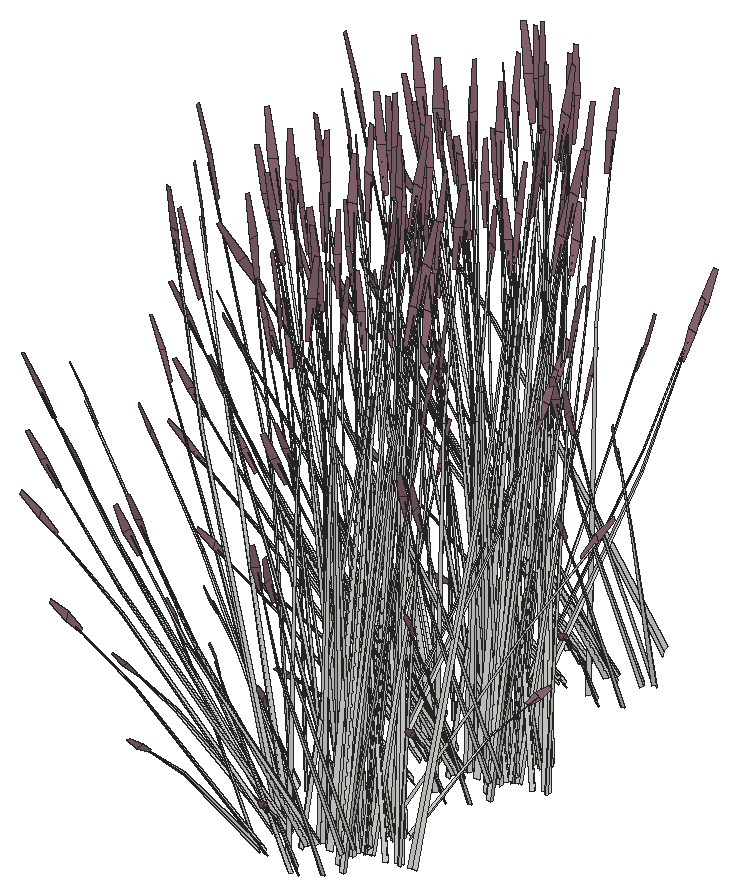
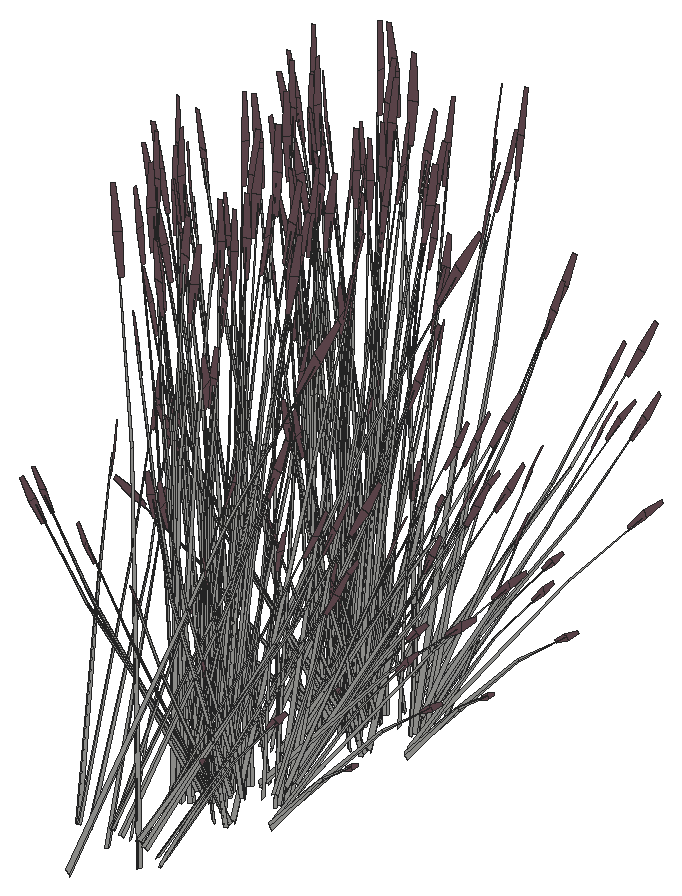
# SketchUp Ruby script. Lengths in inches.
U = 1.inch
M = Sketchup.active_model
def pt(a) = Geom::Point3d.new(a.map { |v| v * U })
def face(e, loops, mat)
  f = e.add_face(loops[0].map { |a| pt(a) })
  loops[1..].each { |l| e.add_face(l.map { |a| pt(a) }).erase! }
  f.material = f.back_material = mat if mat
  f
end
# faces: each face lists its corners as indices into pts; further lists are holes
def faces(e, pts, list, mat = nil) = list.each { |f| face(e, (f[0].is_a?(Array) ? f : [f]).map { |l| l.map { |i| pts[i] } }, mat) }
# xy, xz, yz: faces in a plane at the given z, y or x. An outline is a flat list of corners, or four numbers for a rectangle; further outlines are holes
def ring(l) = l.size == 4 ? [[l[0], l[1]], [l[2], l[1]], [l[2], l[3]], [l[0], l[3]]] : l.each_slice(2).to_a
def flat(e, list, mat, &to3) = list.each { |f| face(e, (f[0].is_a?(Array) ? f : [f]).map { |l| ring(l).map { |u, v| to3.(u, v) } }, mat) }
def xy(e, z, list, mat = nil) = flat(e, list, mat) { |x, y| [x, y, z] }
def xz(e, y, list, mat = nil) = flat(e, list, mat) { |x, z| [x, y, z] }
def yz(e, x, list, mat = nil) = flat(e, list, mat) { |y, z| [x, y, z] }
def lines(e, pts, list) = list.each { |a, b| e.add_line(pt(pts[a]), pt(pts[b])) }
# prism: a flat outline (further loops are holes) pulled along v
def prism(e, loops, v, mat = nil)
  f = face(e, loops, mat); d = Geom::Vector3d.new(v.map { |x| x * U })
  f.pushpull(f.normal.samedirection?(d) ? d.length : -d.length)
end
def box(e, o, s, mat = nil) = prism(e, [[o, [o[0] + s[0], o[1], o[2]], [o[0] + s[0], o[1] + s[1], o[2]], [o[0], o[1] + s[1], o[2]]]], [0, 0, s[2]], mat)
def at(x, y, z, deg = 0) = Geom::Transformation.translation(pt([x, y, z])) * Geom::Transformation.rotation(ORIGIN, Z_AXIS, deg.degrees)
def axes(o, x, y, z) = Geom::Transformation.new([*x, 0, *y, 0, *z, 0, *pt(o).to_a, 1])
def part(name) = M.definitions.add(name)
# library, detail: a bought-in or finely detailed component or shape, given as its bounding box
def library(name, o, s) = part(name).tap { |d| box(d.entities, o, s) }
def detail(e, o, s) = box(e.add_group.entities, o, s)
def put(e, d, t, mat = nil) = e.add_instance(d, t).tap { |i| i.material = mat if mat }
def group(e, t, mat = nil) = e.add_group.tap { |g| g.transformation = t; g.material = mat if mat }.entities
root = M.entities
M.materials.add("LightPink_Translucent").color = [144, 107, 117]
c1 = part("blade")
p = [[2.15,0.21,22],[0,0.17,0],[0.09,0.45,0],[2.18,0.31,22],[2.29,0.31,22],[0.38,0.45,0],
  [2.48,0.24,33],[2.49,0.24,33],[2.48,0.22,33]]
faces(c1.entities,p,[[0,1,2,3],[4,5,2,3],[6,3,4,7],[8,0,3,6]])
c2 = part("seeds")
p = [[0.3,-0.1,1.38],[-0.01,-0.03,1.59],[-0.01,-0.03,0.03],[0.14,-0.07,-0.07],[0.29,-0.03,3],[0.15,0.01,3.11]]
faces(c2.entities,p,[[0,1,2,3],[1,0,4,5]],"LightPink_Translucent")
c3 = part("blade with seeds")
put(c3.entities,c1,at(0,0,0))
put(c3.entities,c2,axes([2.4,0.25,30.99],[1.5799,-0.05474,1.17369],[-0.12525,1.92788,0.29478],[-0.07173,-0.02425,1.56792]))
put(root,c3,axes([23.83,24.14,44.84],[0.42589,0.08502,1.43002],[0.2745,0.86839,-0.30754],[-0.57851,0.16255,0.61141]))
put(root,c3,axes([26.46,19.68,47.23],[-1.22504,-0.02494,-0.71045],[0.08228,-1.05005,0.08574],[-0.51899,-0.11081,1.00501]))
put(root,c3,axes([25.48,19.94,44.84],[0.23927,0.28834,1.43002],[-0.55135,0.78376,-0.30754],[-0.56612,-0.18733,0.61141]))
put(root,c3,axes([25.375,40.2,44.59],[0.42589,0.08502,1.43002],[0.2745,0.86839,-0.30754],[-0.57851,0.16255,0.61141]))
put(root,c3,axes([29.14,37.42,45.34],[0.34834,-0.14982,1.77064],[0.12012,1.04605,0.13857],[-0.75452,0.1388,0.63284]))
put(root,c3,axes([25.19,21.93,46.93],[-0.332,0.94205,-0.51099],[-1.13828,-0.3229,-0.3958],[-0.45829,0.08638,0.97773]))
put(root,c3,axes([26.06,19.9,46.93],[-0.88986,0.68603,-0.51099],[-0.77932,-0.72471,-0.3958],[-0.45212,-0.10438,0.97773]))
put(root,c3,axes([28.01,35.75,46.98],[-1.22504,-0.02494,-0.71045],[0.08228,-1.05005,0.08574],[-0.51899,-0.11081,1.00501]))
put(root,c3,axes([27.02,36,44.59],[0.23927,0.28834,1.43002],[-0.55135,0.78376,-0.30754],[-0.56612,-0.18733,0.61141]))
put(root,c3,axes([22.94,25.96,45.02],[0.51072,-0.46938,1.1486],[0.20153,0.74307,0.84392],[-0.36908,0.13305,0.25299]))
put(root,c3,axes([26.04,37.5625,46.53],[-1.01846,-0.28891,-0.35414],[0.29705,-0.84289,0.4572],[-0.41005,0.07729,0.87481]))
put(root,c3,axes([26.74,37.99,46.68],[-0.332,0.94205,-0.51099],[-1.13828,-0.3229,-0.3958],[-0.45829,0.08638,0.97773]))
put(root,c3,axes([27.6,35.96,46.68],[-0.88986,0.68603,-0.51099],[-0.77932,-0.72471,-0.3958],[-0.45212,-0.10438,0.97773]))
put(root,c3,axes([24.05,20.81,45.02],[0.78239,-0.07411,1.1486],[-0.49629,0.65296,0.84392],[-0.38663,-0.09795,0.25299]))
put(root,c3,axes([24.49,42.02,44.77],[0.51072,-0.46938,1.1486],[0.20153,0.74307,0.84392],[-0.36908,0.13305,0.25299]))
put(root,c3,axes([26.97,54.34,46.53],[-0.69728,-0.64842,-0.35414],[0.79619,-0.61382,0.4572],[-0.40453,-0.09339,0.87481]))
put(root,c3,axes([27.27,35.3125,46.53],[-0.69728,-0.64842,-0.35414],[0.79619,-0.61382,0.4572],[-0.40453,-0.09339,0.87481]))
put(root,c3,axes([26.41,39.99,46.53],[-1.06674,0.14801,-0.35414],[-0.28168,-0.84611,0.4572],[-0.30569,0.22726,0.87481]))
put(root,c3,axes([25.6,36.87,44.77],[0.78239,-0.07411,1.1486],[-0.49629,0.65296,0.84392],[-0.38663,-0.09795,0.25299]))
put(root,c3,axes([25.75,24.03,46.93],[0.31482,0.94565,-0.51099],[-1.19224,0.16542,-0.3958],[-0.34166,0.254,0.97773]))
put(root,c3,axes([28.59,18.45,47.23],[-1.04497,-0.50058,-0.71045],[0.74264,-0.8772,0.08574],[-0.3786,-0.29889,1.00501]))
put(root,c3,axes([28.11,18.47,46.93],[-1.20928,0.24619,-0.51099],[-0.21154,-0.93233,-0.3958],[-0.32481,-0.26718,0.97773]))
put(root,c3,axes([27.75,25.96,44.625],[-0.7662,1.03778,0],[-1.28187,-0.57875,-0.51607],[-0.29196,-0.13181,1.63711]))
put(root,c3,axes([27.29,40.09,46.68],[0.31482,0.94565,-0.51099],[-1.19224,0.16542,-0.3958],[-0.34166,0.254,0.97773]))
put(root,c3,axes([29.84,53.54,46.98],[-1.04497,-0.50058,-0.71045],[0.74264,-0.8772,0.08574],[-0.3786,-0.29889,1.00501]))
put(root,c3,axes([29.35,53.5625,46.68],[-1.20928,0.24619,-0.51099],[-0.21154,-0.93233,-0.3958],[-0.32481,-0.26718,0.97773]))
put(root,c3,axes([30.14,34.51,46.98],[-1.04497,-0.50058,-0.71045],[0.74264,-0.8772,0.08574],[-0.3786,-0.29889,1.00501]))
put(root,c3,axes([26.35,27.46,44.84],[0.38672,-0.16338,1.43002],[0.95481,0.49262,-0.30754],[-0.28419,0.42626,0.61141]))
put(root,c3,axes([29.65,34.53,46.68],[-1.20928,0.24619,-0.51099],[-0.21154,-0.93233,-0.3958],[-0.32481,-0.26718,0.97773]))
put(root,c3,axes([25.8,18.15,44.38],[-0.35352,0.84566,-0.03893],[-1.08806,-0.26014,-0.17649],[-0.1652,-0.13832,0.58215]))
put(root,c3,axes([27.43,17.08,44.84],[-0.07421,0.33879,1.43002],[-1.08488,0.28361,-0.30754],[-0.25359,-0.4379,0.61141]))
put(root,c3,axes([29.29,42.02,44.375],[-0.7662,1.03778,0],[-1.28187,-0.57875,-0.51607],[-0.29196,-0.13181,1.63711]))
put(root,c3,axes([25.22,22.01,44.625],[-1.53239,0,0],[0,-1.1575,-0.51607],[0,-0.26363,1.63711]))
put(root,c3,axes([27.89,43.52,44.59],[0.38672,-0.16338,1.43002],[0.95481,0.49262,-0.30754],[-0.28419,0.42626,0.61141]))
put(root,c3,axes([28.67,52.17,44.59],[-0.07421,0.33879,1.43002],[-1.08488,0.28361,-0.30754],[-0.25359,-0.4379,0.61141]))
put(root,c3,axes([26.4,21.7,44.58],[-1.1399,0.87071,0.30756],[-1.1406,-0.86155,-0.36492],[-0.03981,-0.24727,1.64885]))
put(root,c3,axes([28.97,33.14,44.59],[-0.07421,0.33879,1.43002],[-1.08488,0.28361,-0.30754],[-0.25359,-0.4379,0.61141]))
put(root,c3,axes([29.48,52.875,46.53],[-0.18927,-0.83419,-0.35414],[1.08199,-0.22027,0.4572],[-0.29062,-0.23905,0.87481]))
put(root,c3,axes([27.05,16.54,45.02],[0.63926,0.36046,1.1486],[-0.93099,0.21668,0.84392],[-0.1992,-0.27702,0.25299]))
put(root,c3,axes([27.3,25.32,47.59],[-0.03189,0.95798,-0.7886],[-1.34277,-0.06434,0.09517],[-0.14171,0.40585,1.11556]))
put(root,c3,axes([29.78,33.84,46.53],[-0.18927,-0.83419,-0.35414],[1.08199,-0.22027,0.4572],[-0.29062,-0.23905,0.87481]))
put(root,c3,axes([26.76,38.07,44.375],[-1.53239,0,0],[0,-1.1575,-0.51607],[0,-0.26363,1.63711]))
put(root,c3,axes([27.27,28.01,45.02],[-0.03171,-0.6158,1.1486],[0.7925,0.43922,0.84392],[-0.15586,0.29352,0.25299]))
put(root,c3,axes([28.29,41.95,46.53],[-0.82919,0.54528,-0.35414],[-0.78493,-0.62262,0.4572],[-0.11943,0.31634,0.87481]))
put(root,c3,axes([28.41,25.42,44.73],[1.14694,0.51783,0.49651],[-0.68554,0.92854,0],[-0.26122,-0.11794,1.57504]))
put(root,c3,axes([32.34,59.2,45.33],[1.05902,0.41762,1.51261],[-1.03748,0.89969,0.59816],[-0.46471,-0.53324,1.26806]))
put(root,c3,axes([27.95,37.76,44.33],[-1.1399,0.87071,0.30756],[-1.1406,-0.86155,-0.36492],[-0.03981,-0.24727,1.64885]))
put(root,c3,axes([29.49,23.52,44.69],[0.32481,-1.2272,-0.23429],[1.54007,0.21392,0.51271],[-0.26911,-0.16947,1.5644]))
put(root,c3,axes([28.3,51.625,44.77],[0.63926,0.36046,1.1486],[-0.93099,0.21668,0.84392],[-0.1992,-0.27702,0.25299]))
put(root,c3,axes([32.64,40.17,45.33],[1.05902,0.41762,1.51261],[-1.03748,0.89969,0.59816],[-0.46471,-0.53324,1.26806]))
put(root,c3,axes([30.05,23.81,44.87],[-0.23642,0.92427,0.1448],[-1.15506,-0.16044,-0.41347],[-0.21021,-0.09491,1.26744]))
put(root,c3,axes([28.6,32.6,44.77],[0.63926,0.36046,1.1486],[-0.93099,0.21668,0.84392],[-0.1992,-0.27702,0.25299]))
put(root,c3,axes([26.15,22.18,44.73],[0,1.03566,0.49651],[-1.37109,0,0],[0,-0.23588,1.57504]))
put(root,c3,axes([32.43,26.11,44.44],[-0.75665,-1.04141,-0.05142],[1.28187,-0.57875,0.51607],[-0.31588,0.09915,1.6363]))
put(root,c3,axes([28.84,41.375,47.34],[-0.03189,0.95798,-0.7886],[-1.34277,-0.06434,0.09517],[-0.14171,0.40585,1.11556]))
put(root,c3,axes([28.82,44.07,44.77],[-0.03171,-0.6158,1.1486],[0.7925,0.43922,0.84392],[-0.15586,0.29352,0.25299]))
put(root,c3,axes([27.57,25.63,47.26],[0.87728,0.69587,-0.5672],[-0.92674,0.60943,-0.43934],[-0.13348,0.35356,1.08528]))
put(root,c3,axes([32.74,22.11,45.09],[-0.03348,-0.97511,1.41272],[1.51511,0.25277,0.59816],[-0.35835,0.53357,1.3335]))
put(root,c3,axes([29.95,41.48,44.48],[1.14694,0.51783,0.49651],[-0.68554,0.92854,0],[-0.26122,-0.11794,1.57504]))
put(root,c3,axes([26.62,26.68,45.07],[1.11329,-0.1834,0.06507],[0.25594,0.73887,-0.86304],[-0.07058,0.37403,0.7736]))
put(root,c3,axes([30.79,18.04,46.93],[-1.20468,-0.25962,-0.51099],[0.41292,-0.89013,-0.3958],[-0.11046,-0.35838,0.97773]))
put(root,c3,axes([31.59,39.87,44.62],[-0.23642,0.92427,0.1448],[-1.15506,-0.16044,-0.41347],[-0.21021,-0.09491,1.26744]))
put(root,c3,axes([27.69,38.25,44.48],[0,1.03566,0.49651],[-1.37109,0,0],[0,-0.23588,1.57504]))
put(root,c3,axes([33.97,42.17,44.19],[-0.75665,-1.04141,-0.05142],[1.28187,-0.57875,0.51607],[-0.31588,0.09915,1.6363]))
put(root,c3,axes([30.01,17.07,44.38],[-0.84686,0.59414,-0.03893],[-0.77596,-0.65071,-0.17649],[-0.05463,-0.18438,0.58215]))
put(root,c3,axes([29.67,22.93,44.61],[1.54892,0.2182,0.45755],[-0.31522,1.23236,0.17955],[-0.22636,-0.119,1.58856]))
put(root,c3,axes([29.12,41.69,47],[0.87728,0.69587,-0.5672],[-0.92674,0.60943,-0.43934],[-0.13348,0.35356,1.08528]))
put(root,c3,axes([34.28,38.17,44.84],[-0.03348,-0.97511,1.41272],[1.51511,0.25277,0.59816],[-0.35835,0.53357,1.3335]))
put(root,c3,axes([29.27,22.7,44.97],[-0.59459,0.93321,0.44739],[-1.23546,-0.44912,-0.21531],[0,-0.21512,1.43643]))
put(root,c3,axes([31.23,18.21,47.23],[-0.5849,-0.8421,-0.71045],[1.20401,-0.4693,0.08574],[-0.13677,-0.40688,1.00501]))
put(root,c3,axes([32.04,53.13,46.68],[-1.20468,-0.25962,-0.51099],[0.41292,-0.89013,-0.3958],[-0.11046,-0.35838,0.97773]))
put(root,c3,axes([28.16,42.74,44.82],[1.11329,-0.1834,0.06507],[0.25594,0.73887,-0.86304],[-0.07058,0.37403,0.7736]))
put(root,c3,axes([28.84,24.9,44.72],[1.31687,-0.27488,0.17642],[0.32517,1.02297,0.35086],[-0.11745,-0.14905,1.60407]))
put(root,c3,axes([32.34,34.1,46.68],[-1.20468,-0.25962,-0.51099],[0.41292,-0.89013,-0.3958],[-0.11046,-0.35838,0.97773]))
put(root,c3,axes([30.53,25.06,44.45],[-1.23546,-0.46496,0],[0.59459,-0.96613,0],[0,0,1.62707]))
put(root,c3,axes([33.39,26.22,44.625],[0.7662,1.03778,0],[-1.28187,0.57875,-0.51607],[-0.29196,0.13181,1.63711]))
put(root,c3,axes([31.21,38.99,44.36],[1.54892,0.2182,0.45755],[-0.31522,1.23236,0.17955],[-0.22636,-0.119,1.58856]))
put(root,c3,axes([32.48,53.3,46.98],[-0.5849,-0.8421,-0.71045],[1.20401,-0.4693,0.08574],[-0.13677,-0.40688,1.00501]))
put(root,c3,axes([32.76,24.95,44.72],[0.35402,-1.02926,0.17642],[1.29548,0.29127,0.35086],[-0.22379,0.00501,1.60407]))
put(root,c3,axes([32.16,23.59,44.87],[0.90538,0.62224,0.1448],[-0.75521,0.70202,-0.41347],[-0.21021,0.09491,1.26744]))
put(root,c3,axes([30.8125,38.77,44.72],[-0.59459,0.93321,0.44739],[-1.23546,-0.44912,-0.21531],[0,-0.21512,1.43643]))
put(root,c3,axes([32.77,34.27,46.98],[-0.5849,-0.8421,-0.71045],[1.20401,-0.4693,0.08574],[-0.13677,-0.40688,1.00501]))
put(root,c3,axes([31.84,22.82,44.55],[-1.1399,-0.8914,-0.06131],[1.1406,-0.89194,0],[-0.03981,-0.03113,1.75571]))
put(root,c3,axes([32.14,23.13,44.97],[1.33077,-0.06393,0.44739],[0.12035,1.06125,-0.21531],[-0.23824,0.10756,1.43643]))
put(root,c3,axes([32.46,25.57,44.58],[1.53422,0.33662,0.30756],[-0.38383,1.20322,-0.36492],[-0.25393,0.15059,1.64885]))
put(root,c3,axes([33.12,25.5,44.73],[1.14694,-0.51783,0.49651],[0.68554,0.92854,0],[-0.26122,0.11794,1.57504]))
put(root,c3,axes([30.38,40.96,44.47],[1.31687,-0.27488,0.17642],[0.32517,1.02297,0.35086],[-0.11745,-0.14905,1.60407]))
put(root,c3,axes([29.54,21.79,44.61],[0.53281,1.15808,0.45755],[-1.52239,0.4027,0.17955],[0.01861,-0.2128,1.58856]))
put(root,c3,axes([32.08,41.12,44.2],[-1.23546,-0.46496,0],[0.59459,-0.96613,0],[0,0,1.62707]))
put(root,c3,axes([30.8125,24.66,44.45],[-0.39985,-0.89288,0],[1.1418,-0.31268,0],[0,0,1.54371]))
put(root,c3,axes([34.93,42.28,44.375],[0.7662,1.03778,0],[-1.28187,0.57875,-0.51607],[-0.29196,0.13181,1.63711]))
put(root,c3,axes([34.3,41.01,44.47],[0.35402,-1.02926,0.17642],[1.29548,0.29127,0.35086],[-0.22379,0.00501,1.60407]))
put(root,c3,axes([33.7,39.65,44.62],[0.90538,0.62224,0.1448],[-0.75521,0.70202,-0.41347],[-0.21021,0.09491,1.26744]))
put(root,c3,axes([33.38,38.88,44.3],[-1.1399,-0.8914,-0.06131],[1.1406,-0.89194,0],[-0.03981,-0.03113,1.75571]))
put(root,c3,axes([33.68,39.19,44.72],[1.33077,-0.06393,0.44739],[0.12035,1.06125,-0.21531],[-0.23824,0.10756,1.43643]))
put(root,c3,axes([34,41.63,44.33],[1.53422,0.33662,0.30756],[-0.38383,1.20322,-0.36492],[-0.25393,0.15059,1.64885]))
put(root,c3,axes([32.59,52.58,46.53],[0.36946,-0.79643,-0.35414],[1.07787,0.23229,0.4572],[-0.09883,-0.32066,0.87481]))
put(root,c3,axes([34.78,22.33,44.72],[-0.96285,-0.75439,0.17642],[0.97031,-0.7317,0.35086],[-0.10634,0.15406,1.60407]))
put(root,c3,axes([34.66,41.56,44.48],[1.14694,-0.51783,0.49651],[0.68554,0.92854,0],[-0.26122,0.11794,1.57504]))
put(root,c3,axes([31.45,21.89,44.46],[0,-1.19833,0],[1.53239,0,0],[0,0,1.79456]))
put(root,c3,axes([32.89,33.55,46.53],[0.36946,-0.79643,-0.35414],[1.07787,0.23229,0.4572],[-0.09883,-0.32066,0.87481]))
put(root,c3,axes([31.08,37.85,44.36],[0.53281,1.15808,0.45755],[-1.52239,0.4027,0.17955],[0.01861,-0.2128,1.58856]))
put(root,c3,axes([30.03,22.11,44.68],[1.3808,0.50196,0.24065],[-0.66454,1.04299,0.50002],[0,-0.24043,1.60543]))
put(root,c3,axes([32.22,22.37,44.54],[0,1.19774,-0.05637],[-1.53239,0,0],[0,0.03764,1.79368]))
put(root,c3,axes([29.58,21.41,44.97],[-1.33077,0.06393,0.44739],[-0.12035,-1.06125,-0.21531],[0.23824,-0.10756,1.43643]))
put(root,c3,axes([32.36,40.72,44.2],[-0.39985,-0.89288,0],[1.1418,-0.31268,0],[0,0,1.54371]))
put(root,c3,axes([31.17,42.91,46.53],[-0.36946,0.79643,-0.35414],[-1.07787,-0.23229,0.4572],[0.09883,0.32066,0.87481]))
put(root,c3,axes([28.96,19.59,44.72],[-0.35402,1.02926,0.17642],[-1.29548,-0.29127,0.35086],[0.22379,-0.00501,1.60407]))
put(root,c3,axes([31.49,24.6875,44.54],[0.53281,1.18979,-0.06012],[-1.52239,0.41691,0],[0.01861,0.04155,1.72173]))
put(root,c3,axes([28.33,18.32,44.625],[-0.7662,-1.03778,0],[1.28187,-0.57875,-0.51607],[0.29196,-0.13181,1.63711]))
put(root,c3,axes([29.73,26.14,47.23],[0.5849,0.8421,-0.71045],[-1.20401,0.4693,0.08574],[0.13677,0.40688,1.00501]))
put(root,c3,axes([35.89,23.125,44.45],[-1.53164,-0.00828,-0.04976],[0,-1.1575,0.49943],[-0.04813,0.2635,1.58352]))
put(root,c3,axes([32.88,19.64,44.72],[-1.31687,0.27488,0.17642],[-0.32517,-1.02297,0.35086],[0.11745,0.14905,1.60407]))
put(root,c3,axes([36.32,38.39,44.47],[-0.96285,-0.75439,0.17642],[0.97031,-0.7317,0.35086],[-0.10634,0.15406,1.60407]))
put(root,c3,axes([31.54,15.81,45.02],[0.15721,0.60392,1.1486],[-0.87211,-0.33448,0.84392],[0.09385,-0.30923,0.25299]))
put(root,c3,axes([33,37.95,44.21],[0,-1.19833,0],[1.53239,0,0],[0,0,1.79456]))
put(root,c3,axes([31.57,38.17,44.43],[1.3808,0.50196,0.24065],[-0.66454,1.04299,0.50002],[0,-0.24043,1.60543]))
put(root,c3,axes([30.73,21.14,44.61],[-1.01611,0.93987,0.45755],[-1.20717,-0.82966,0.17955],[0.24496,-0.0938,1.58856]))
put(root,c3,axes([33.77,38.43,44.29],[0,1.19774,-0.05637],[-1.53239,0,0],[0,0.03764,1.79368]))
put(root,c3,axes([31.125,37.47,44.72],[-1.33077,0.06393,0.44739],[-0.12035,-1.06125,-0.21531],[0.23824,-0.10756,1.43643]))
put(root,c3,axes([32.46,22.62,44.47],[0.85545,0.66896,0],[-0.85545,0.66896,0],[0,0,1.69266]))
put(root,c3,axes([32.45,21.84,44.97],[0.59459,-0.93321,0.44739],[1.23546,0.44912,-0.21531],[0,0.21512,1.43643]))
put(root,c3,axes([31.93,25.08,44.45],[1.23546,0.46496,0],[-0.59459,0.96613,0],[0,0,1.74954]))
put(root,c3,axes([30.51,35.65,44.47],[-0.35402,1.02926,0.17642],[-1.29548,-0.29127,0.35086],[0.22379,-0.00501,1.60407]))
put(root,c3,axes([33.03,40.75,44.29],[0.53281,1.18979,-0.06012],[-1.52239,0.41691,0],[0.01861,0.04155,1.72173]))
put(root,c3,axes([30.17,26.31,46.93],[1.20468,0.25962,-0.51099],[-0.41292,0.89013,-0.3958],[0.11046,0.35838,0.97773]))
put(root,c3,axes([32.05,21.61,44.63],[-1.54892,-0.2182,0.49198],[0.31522,-1.23236,0.19306],[0.22636,0.119,1.70813]))
put(root,c3,axes([29.57,53.41,44.375],[-0.7662,-1.03778,0],[1.28187,-0.57875,-0.51607],[0.29196,-0.13181,1.63711]))
put(root,c3,axes([29.87,34.38,44.375],[-0.7662,-1.03778,0],[1.28187,-0.57875,-0.51607],[0.29196,-0.13181,1.63711]))
put(root,c3,axes([31.28,42.2,46.98],[0.5849,0.8421,-0.71045],[-1.20401,0.4693,0.08574],[0.13677,0.40688,1.00501]))
put(root,c3,axes([37.43,39.1875,44.2],[-1.53164,-0.00828,-0.04976],[0,-1.1575,0.49943],[-0.04813,0.2635,1.58352]))
put(root,c3,axes([32.49,22.16,44.46],[1.37109,0,0],[0,1.07219,0],[0,0,1.78407]))
put(root,c3,axes([32.78,50.9,44.77],[0.15721,0.60392,1.1486],[-0.87211,-0.33448,0.84392],[0.09385,-0.30923,0.25299]))
put(root,c3,axes([34.43,35.7,44.47],[-1.31687,0.27488,0.17642],[-0.32517,-1.02297,0.35086],[0.11745,0.14905,1.60407]))
put(root,c3,axes([31.17,20.98,44.97],[-0.73619,-0.86927,0.44739],[1.11511,-0.61213,-0.21531],[0.23824,0.10756,1.43643]))
put(root,c3,axes([32.97,22.05,44.87],[1.1418,-0.30203,0.1448],[0.39985,0.86246,-0.41347],[0,0.18981,1.26744]))
put(root,c3,axes([33.39,18.71,46.93],[-0.87728,-0.69587,-0.51099],[0.92674,-0.60943,-0.3958],[0.13348,-0.35356,0.97773]))
put(root,c3,axes([33.08,31.87,44.77],[0.15721,0.60392,1.1486],[-0.87211,-0.33448,0.84392],[0.09385,-0.30923,0.25299]))
put(root,c3,axes([32.27,37.2,44.36],[-1.01611,0.93987,0.45755],[-1.20717,-0.82966,0.17955],[0.24496,-0.0938,1.58856]))
put(root,c3,axes([34.01,38.68,44.21],[0.85545,0.66896,0],[-0.85545,0.66896,0],[0,0,1.69266]))
put(root,c3,axes([33.99,37.9,44.72],[0.59459,-0.93321,0.44739],[1.23546,0.44912,-0.21531],[0,0.21512,1.43643]))
put(root,c3,axes([33.48,41.14,44.2],[1.23546,0.46496,0],[-0.59459,0.96613,0],[0,0,1.74954]))
put(root,c3,axes([31.72,42.37,46.68],[1.20468,0.25962,-0.51099],[-0.41292,0.89013,-0.3958],[0.11046,0.35838,0.97773]))
put(root,c3,axes([33.59,37.67,44.38],[-1.54892,-0.2182,0.49198],[0.31522,-1.23236,0.19306],[0.22636,0.119,1.70813]))
put(root,c3,axes([32.82,17.48,44.84],[-0.34835,0.20963,1.43002],[-1.04325,-0.36691,-0.30754],[0.19338,-0.4563,0.61141]))
put(root,c3,axes([35.57,22.36,44.73],[0,-1.03566,0.49651],[1.37109,0,0],[0,0.23588,1.57504]))
put(root,c3,axes([34.64,53.8,46.68],[-0.87728,-0.69587,-0.51099],[0.92674,-0.60943,-0.3958],[0.13348,-0.35356,0.97773]))
put(root,c3,axes([34.04,38.22,44.21],[1.37109,0,0],[0,1.07219,0],[0,0,1.78407]))
put(root,c3,axes([31.67,20.73,44.87],[0.23642,-0.92427,0.1448],[1.15506,0.16044,-0.41347],[0.21021,0.09491,1.26744]))
put(root,c3,axes([32.72,37.04,44.72],[-0.73619,-0.86927,0.44739],[1.11511,-0.61213,-0.21531],[0.23824,0.10756,1.43643]))
put(root,c3,axes([34.51,38.11,44.62],[1.1418,-0.30203,0.1448],[0.39985,0.86246,-0.41347],[0,0.18981,1.26744]))
put(root,c3,axes([34.9375,34.77,46.68],[-0.87728,-0.69587,-0.51099],[0.92674,-0.60943,-0.3958],[0.13348,-0.35356,0.97773]))
put(root,c3,axes([33.31,19.12,44.73],[-1.14694,-0.51783,0.49651],[0.68554,-0.92854,0],[0.26122,0.11794,1.57504]))
put(root,c3,axes([33.67,19.03,47.23],[0.03189,-0.95798,-0.71045],[1.34277,0.06434,0.08574],[0.14171,-0.40585,1.00501]))
put(root,c3,axes([34.06,52.57,44.59],[-0.34835,0.20963,1.43002],[-1.04325,-0.36691,-0.30754],[0.19338,-0.4563,0.61141]))
put(root,c3,axes([34.36,33.54,44.59],[-0.34835,0.20963,1.43002],[-1.04325,-0.36691,-0.30754],[0.19338,-0.4563,0.61141]))
put(root,c3,axes([37.12,38.42,44.48],[0,-1.03566,0.49651],[1.37109,0,0],[0,0.23588,1.57504]))
put(root,c3,axes([33.21,36.79,44.62],[0.23642,-0.92427,0.1448],[1.15506,0.16044,-0.41347],[0.21021,0.09491,1.26744]))
put(root,c3,axes([34.91,54.12,46.98],[0.03189,-0.95798,-0.71045],[1.34277,0.06434,0.08574],[0.14171,-0.40585,1.00501]))
put(root,c3,axes([34.42,25.47,45.02],[-0.69001,-0.29779,1.1486],[0.89096,-0.30257,0.84392],[0.24031,0.2563,0.25299]))
put(root,c3,axes([31.96,25.15,44.84],[0.02163,-0.34331,1.43002],[1.03345,-0.38348,-0.30754],[0.31903,0.4109,0.61141]))
put(root,c3,axes([34.85,35.18,44.48],[-1.14694,-0.51783,0.49651],[0.68554,-0.92854,0],[0.26122,0.11794,1.57504]))
put(root,c3,axes([35.21,35.09,46.98],[0.03189,-0.95798,-0.71045],[1.34277,0.06434,0.08574],[0.14171,-0.40585,1.00501]))
put(root,c3,axes([36.5,22.53,44.63],[1.53239,0,0],[0,1.1575,-0.51607],[0,0.26363,1.63711]))
put(root,c3,axes([35.46,53.55,46.53],[0.82919,-0.54528,-0.35414],[0.78493,0.62262,0.4572],[0.11943,-0.31634,0.87481]))
